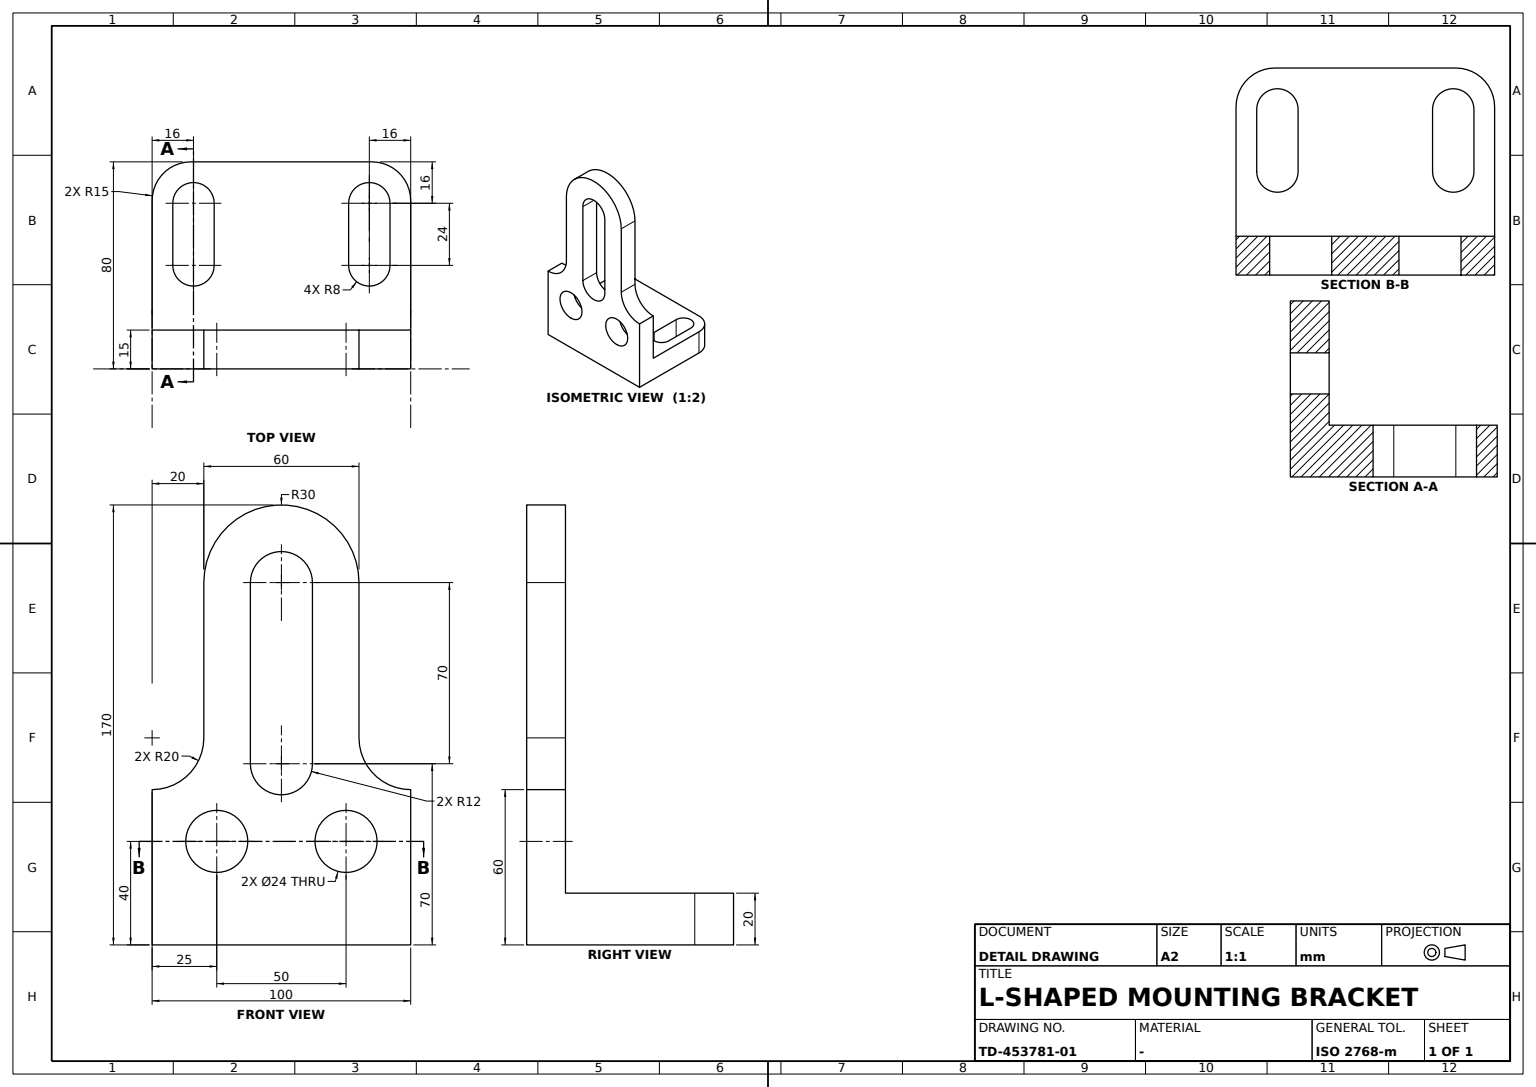
ISO-10303-21;
HEADER;
FILE_DESCRIPTION((''),'2;1');
FILE_NAME('','',(''),(''),'','','');
FILE_SCHEMA(('AUTOMOTIVE_DESIGN'));
ENDSEC;
DATA;
#1=APPLICATION_CONTEXT('');
#2=PRODUCT_CONTEXT('',#1,'mechanical');
#3=PRODUCT('','','',(#2));
#4=PRODUCT_DEFINITION_FORMATION('','',#3);
#5=PRODUCT_DEFINITION_CONTEXT('',#1,'design');
#6=PRODUCT_DEFINITION('','',#4,#5);
#7=PRODUCT_DEFINITION_SHAPE('','',#6);
#8=(LENGTH_UNIT()NAMED_UNIT(*)SI_UNIT(.MILLI.,.METRE.));
#9=(NAMED_UNIT(*)PLANE_ANGLE_UNIT()SI_UNIT($,.RADIAN.));
#10=(NAMED_UNIT(*)SI_UNIT($,.STERADIAN.)SOLID_ANGLE_UNIT());
#11=UNCERTAINTY_MEASURE_WITH_UNIT(LENGTH_MEASURE(0.005),#8,'distance_accuracy_value','');
#12=(GEOMETRIC_REPRESENTATION_CONTEXT(3)GLOBAL_UNCERTAINTY_ASSIGNED_CONTEXT((#11))GLOBAL_UNIT_ASSIGNED_CONTEXT((#8,#9,#10))REPRESENTATION_CONTEXT('',''));
#13=CARTESIAN_POINT('',(-12.,0.,130.));
#14=VERTEX_POINT('',#13);
#15=CARTESIAN_POINT('',(-12.,0.,60.));
#16=VERTEX_POINT('',#15);
#17=DIRECTION('',(0.,0.,-1.));
#18=VECTOR('',#17,1000.);
#19=LINE('',#13,#18);
#20=EDGE_CURVE('',#14,#16,#19,.T.);
#21=ORIENTED_EDGE('',*,*,#20,.T.);
#22=CARTESIAN_POINT('',(-12.,15.,60.));
#23=VERTEX_POINT('',#22);
#24=CARTESIAN_POINT('',(-12.,7.5,60.));
#25=DIRECTION('',(0.,-1.,0.));
#26=VECTOR('',#25,1000.);
#27=LINE('',#24,#26);
#28=EDGE_CURVE('',#16,#23,#27,.F.);
#29=ORIENTED_EDGE('',*,*,#28,.T.);
#30=CARTESIAN_POINT('',(-12.,15.,130.));
#31=VERTEX_POINT('',#30);
#32=LINE('',#30,#18);
#33=EDGE_CURVE('',#31,#23,#32,.T.);
#34=ORIENTED_EDGE('',*,*,#33,.F.);
#35=CARTESIAN_POINT('',(-12.,7.5,130.));
#36=LINE('',#35,#26);
#37=EDGE_CURVE('',#14,#31,#36,.F.);
#38=ORIENTED_EDGE('',*,*,#37,.F.);
#39=EDGE_LOOP('',(#21,#29,#34,#38));
#40=FACE_BOUND('',#39,.T.);
#41=DIRECTION('',(1.,0.,0.));
#42=AXIS2_PLACEMENT_3D('',#13,#41,#17);
#43=PLANE('',#42);
#44=ADVANCED_FACE('',(#40),#43,.T.);
#45=CARTESIAN_POINT('',(26.,40.,-10.));
#46=VERTEX_POINT('',#45);
#47=CARTESIAN_POINT('',(42.,40.,-10.));
#48=VERTEX_POINT('',#47);
#49=CARTESIAN_POINT('',(34.,40.,-10.));
#50=DIRECTION('',(0.,0.,1.));
#51=AXIS2_PLACEMENT_3D('',#49,#50,#41);
#52=CIRCLE('',#51,8.);
#53=EDGE_CURVE('',#46,#48,#52,.T.);
#54=ORIENTED_EDGE('',*,*,#53,.T.);
#55=CARTESIAN_POINT('',(42.,64.,-10.));
#56=VERTEX_POINT('',#55);
#57=CARTESIAN_POINT('',(42.,0.,-10.));
#58=DIRECTION('',(0.,1.,0.));
#59=VECTOR('',#58,1000.);
#60=LINE('',#57,#59);
#61=EDGE_CURVE('',#48,#56,#60,.T.);
#62=ORIENTED_EDGE('',*,*,#61,.T.);
#63=CARTESIAN_POINT('',(26.,64.,-10.));
#64=VERTEX_POINT('',#63);
#65=CARTESIAN_POINT('',(34.,64.,-10.));
#66=AXIS2_PLACEMENT_3D('',#65,#50,#41);
#67=CIRCLE('',#66,8.);
#68=EDGE_CURVE('',#56,#64,#67,.T.);
#69=ORIENTED_EDGE('',*,*,#68,.T.);
#70=CARTESIAN_POINT('',(26.,0.,-10.));
#71=LINE('',#70,#59);
#72=EDGE_CURVE('',#46,#64,#71,.T.);
#73=ORIENTED_EDGE('',*,*,#72,.F.);
#74=EDGE_LOOP('',(#54,#62,#69,#73));
#75=FACE_BOUND('',#74,.T.);
#76=CARTESIAN_POINT('',(-50.,0.,-10.));
#77=VERTEX_POINT('',#76);
#78=CARTESIAN_POINT('',(-50.,65.,-10.));
#79=VERTEX_POINT('',#78);
#80=LINE('',#76,#59);
#81=EDGE_CURVE('',#77,#79,#80,.T.);
#82=ORIENTED_EDGE('',*,*,#81,.T.);
#83=CARTESIAN_POINT('',(-35.,80.,-10.));
#84=VERTEX_POINT('',#83);
#85=CARTESIAN_POINT('',(-35.,65.,-10.));
#86=AXIS2_PLACEMENT_3D('',#85,#50,#41);
#87=CIRCLE('',#86,15.);
#88=EDGE_CURVE('',#84,#79,#87,.T.);
#89=ORIENTED_EDGE('',*,*,#88,.F.);
#90=CARTESIAN_POINT('',(35.,80.,-10.));
#91=VERTEX_POINT('',#90);
#92=CARTESIAN_POINT('',(0.,80.,-10.));
#93=DIRECTION('',(-1.,0.,0.));
#94=VECTOR('',#93,1000.);
#95=LINE('',#92,#94);
#96=EDGE_CURVE('',#91,#84,#95,.T.);
#97=ORIENTED_EDGE('',*,*,#96,.F.);
#98=CARTESIAN_POINT('',(50.,65.,-10.));
#99=VERTEX_POINT('',#98);
#100=CARTESIAN_POINT('',(35.,65.,-10.));
#101=AXIS2_PLACEMENT_3D('',#100,#50,#41);
#102=CIRCLE('',#101,15.);
#103=EDGE_CURVE('',#99,#91,#102,.T.);
#104=ORIENTED_EDGE('',*,*,#103,.F.);
#105=CARTESIAN_POINT('',(50.,0.,-10.));
#106=VERTEX_POINT('',#105);
#107=LINE('',#105,#26);
#108=EDGE_CURVE('',#99,#106,#107,.T.);
#109=ORIENTED_EDGE('',*,*,#108,.T.);
#110=CARTESIAN_POINT('',(0.,0.,-10.));
#111=VECTOR('',#41,1000.);
#112=LINE('',#110,#111);
#113=EDGE_CURVE('',#77,#106,#112,.T.);
#114=ORIENTED_EDGE('',*,*,#113,.F.);
#115=EDGE_LOOP('',(#82,#89,#97,#104,#109,#114));
#116=FACE_BOUND('',#115,.T.);
#117=CARTESIAN_POINT('',(-26.,40.,-10.));
#118=VERTEX_POINT('',#117);
#119=CARTESIAN_POINT('',(-26.,64.,-10.));
#120=VERTEX_POINT('',#119);
#121=CARTESIAN_POINT('',(-26.,0.,-10.));
#122=LINE('',#121,#59);
#123=EDGE_CURVE('',#118,#120,#122,.T.);
#124=ORIENTED_EDGE('',*,*,#123,.T.);
#125=CARTESIAN_POINT('',(-42.,64.,-10.));
#126=VERTEX_POINT('',#125);
#127=CARTESIAN_POINT('',(-34.,64.,-10.));
#128=AXIS2_PLACEMENT_3D('',#127,#50,#41);
#129=CIRCLE('',#128,8.);
#130=EDGE_CURVE('',#120,#126,#129,.T.);
#131=ORIENTED_EDGE('',*,*,#130,.T.);
#132=CARTESIAN_POINT('',(-42.,40.,-10.));
#133=VERTEX_POINT('',#132);
#134=CARTESIAN_POINT('',(-42.,0.,-10.));
#135=LINE('',#134,#59);
#136=EDGE_CURVE('',#133,#126,#135,.T.);
#137=ORIENTED_EDGE('',*,*,#136,.F.);
#138=CARTESIAN_POINT('',(-34.,40.,-10.));
#139=AXIS2_PLACEMENT_3D('',#138,#50,#41);
#140=CIRCLE('',#139,8.);
#141=EDGE_CURVE('',#133,#118,#140,.T.);
#142=ORIENTED_EDGE('',*,*,#141,.T.);
#143=EDGE_LOOP('',(#124,#131,#137,#142));
#144=FACE_BOUND('',#143,.T.);
#145=AXIS2_PLACEMENT_3D('',#110,#50,#58);
#146=PLANE('',#145);
#147=ADVANCED_FACE('',(#75,#116,#144),#146,.F.);
#148=ORIENTED_EDGE('',*,*,#37,.T.);
#149=CARTESIAN_POINT('',(12.,15.,130.));
#150=VERTEX_POINT('',#149);
#151=CARTESIAN_POINT('',(0.,15.,130.));
#152=AXIS2_PLACEMENT_3D('',#151,#25,#17);
#153=CIRCLE('',#152,12.);
#154=EDGE_CURVE('',#150,#31,#153,.T.);
#155=ORIENTED_EDGE('',*,*,#154,.F.);
#156=CARTESIAN_POINT('',(12.,0.,130.));
#157=VERTEX_POINT('',#156);
#158=CARTESIAN_POINT('',(12.,7.5,130.));
#159=LINE('',#158,#26);
#160=EDGE_CURVE('',#157,#150,#159,.F.);
#161=ORIENTED_EDGE('',*,*,#160,.F.);
#162=CARTESIAN_POINT('',(0.,0.,130.));
#163=AXIS2_PLACEMENT_3D('',#162,#25,#17);
#164=CIRCLE('',#163,12.);
#165=EDGE_CURVE('',#157,#14,#164,.T.);
#166=ORIENTED_EDGE('',*,*,#165,.T.);
#167=EDGE_LOOP('',(#148,#155,#161,#166));
#168=FACE_BOUND('',#167,.T.);
#169=CARTESIAN_POINT('',(0.,7.5,130.));
#170=AXIS2_PLACEMENT_3D('',#169,#25,#41);
#171=CYLINDRICAL_SURFACE('',#170,12.);
#172=ADVANCED_FACE('',(#168),#171,.F.);
#173=CARTESIAN_POINT('',(-26.,40.,10.));
#174=VERTEX_POINT('',#173);
#175=CARTESIAN_POINT('',(-26.,40.,0.));
#176=VECTOR('',#50,1000.);
#177=LINE('',#175,#176);
#178=EDGE_CURVE('',#118,#174,#177,.T.);
#179=ORIENTED_EDGE('',*,*,#178,.F.);
#180=ORIENTED_EDGE('',*,*,#141,.F.);
#181=CARTESIAN_POINT('',(-42.,40.,10.));
#182=VERTEX_POINT('',#181);
#183=CARTESIAN_POINT('',(-42.,40.,0.));
#184=LINE('',#183,#176);
#185=EDGE_CURVE('',#133,#182,#184,.T.);
#186=ORIENTED_EDGE('',*,*,#185,.T.);
#187=CARTESIAN_POINT('',(-34.,40.,10.));
#188=AXIS2_PLACEMENT_3D('',#187,#50,#41);
#189=CIRCLE('',#188,8.);
#190=EDGE_CURVE('',#182,#174,#189,.T.);
#191=ORIENTED_EDGE('',*,*,#190,.T.);
#192=EDGE_LOOP('',(#179,#180,#186,#191));
#193=FACE_BOUND('',#192,.T.);
#194=CARTESIAN_POINT('',(-34.,40.,0.));
#195=AXIS2_PLACEMENT_3D('',#194,#50,#58);
#196=CYLINDRICAL_SURFACE('',#195,8.);
#197=ADVANCED_FACE('',(#193),#196,.F.);
#198=CARTESIAN_POINT('',(42.,40.,10.));
#199=VERTEX_POINT('',#198);
#200=CARTESIAN_POINT('',(42.,40.,0.));
#201=LINE('',#200,#176);
#202=EDGE_CURVE('',#48,#199,#201,.T.);
#203=ORIENTED_EDGE('',*,*,#202,.F.);
#204=ORIENTED_EDGE('',*,*,#53,.F.);
#205=CARTESIAN_POINT('',(26.,40.,10.));
#206=VERTEX_POINT('',#205);
#207=CARTESIAN_POINT('',(26.,40.,0.));
#208=LINE('',#207,#176);
#209=EDGE_CURVE('',#46,#206,#208,.T.);
#210=ORIENTED_EDGE('',*,*,#209,.T.);
#211=CARTESIAN_POINT('',(34.,40.,10.));
#212=AXIS2_PLACEMENT_3D('',#211,#50,#41);
#213=CIRCLE('',#212,8.);
#214=EDGE_CURVE('',#206,#199,#213,.T.);
#215=ORIENTED_EDGE('',*,*,#214,.T.);
#216=EDGE_LOOP('',(#203,#204,#210,#215));
#217=FACE_BOUND('',#216,.T.);
#218=CARTESIAN_POINT('',(34.,40.,0.));
#219=AXIS2_PLACEMENT_3D('',#218,#50,#58);
#220=CYLINDRICAL_SURFACE('',#219,8.);
#221=ADVANCED_FACE('',(#217),#220,.F.);
#222=CARTESIAN_POINT('',(-30.,0.,70.));
#223=VERTEX_POINT('',#222);
#224=CARTESIAN_POINT('',(-30.,0.,130.));
#225=VERTEX_POINT('',#224);
#226=CARTESIAN_POINT('',(-30.,0.,50.));
#227=LINE('',#226,#176);
#228=EDGE_CURVE('',#223,#225,#227,.T.);
#229=ORIENTED_EDGE('',*,*,#228,.T.);
#230=CARTESIAN_POINT('',(-30.,15.,130.));
#231=VERTEX_POINT('',#230);
#232=CARTESIAN_POINT('',(-30.,7.5,130.));
#233=LINE('',#232,#26);
#234=EDGE_CURVE('',#225,#231,#233,.F.);
#235=ORIENTED_EDGE('',*,*,#234,.T.);
#236=CARTESIAN_POINT('',(-30.,15.,70.));
#237=VERTEX_POINT('',#236);
#238=CARTESIAN_POINT('',(-30.,15.,50.));
#239=LINE('',#238,#176);
#240=EDGE_CURVE('',#237,#231,#239,.T.);
#241=ORIENTED_EDGE('',*,*,#240,.F.);
#242=CARTESIAN_POINT('',(-30.,7.5,70.));
#243=LINE('',#242,#26);
#244=EDGE_CURVE('',#223,#237,#243,.F.);
#245=ORIENTED_EDGE('',*,*,#244,.F.);
#246=EDGE_LOOP('',(#229,#235,#241,#245));
#247=FACE_BOUND('',#246,.T.);
#248=AXIS2_PLACEMENT_3D('',#226,#93,#50);
#249=PLANE('',#248);
#250=ADVANCED_FACE('',(#247),#249,.T.);
#251=CARTESIAN_POINT('',(30.,0.,130.));
#252=VERTEX_POINT('',#251);
#253=CARTESIAN_POINT('',(30.,15.,130.));
#254=VERTEX_POINT('',#253);
#255=CARTESIAN_POINT('',(30.,7.5,130.));
#256=LINE('',#255,#26);
#257=EDGE_CURVE('',#252,#254,#256,.F.);
#258=ORIENTED_EDGE('',*,*,#257,.F.);
#259=CARTESIAN_POINT('',(30.,0.,70.));
#260=VERTEX_POINT('',#259);
#261=LINE('',#251,#18);
#262=EDGE_CURVE('',#252,#260,#261,.T.);
#263=ORIENTED_EDGE('',*,*,#262,.T.);
#264=CARTESIAN_POINT('',(30.,15.,70.));
#265=VERTEX_POINT('',#264);
#266=CARTESIAN_POINT('',(30.,7.5,70.));
#267=LINE('',#266,#59);
#268=EDGE_CURVE('',#260,#265,#267,.T.);
#269=ORIENTED_EDGE('',*,*,#268,.T.);
#270=LINE('',#253,#18);
#271=EDGE_CURVE('',#254,#265,#270,.T.);
#272=ORIENTED_EDGE('',*,*,#271,.F.);
#273=EDGE_LOOP('',(#258,#263,#269,#272));
#274=FACE_BOUND('',#273,.T.);
#275=AXIS2_PLACEMENT_3D('',#251,#41,#17);
#276=PLANE('',#275);
#277=ADVANCED_FACE('',(#274),#276,.T.);
#278=CARTESIAN_POINT('',(12.,0.,60.));
#279=VERTEX_POINT('',#278);
#280=CARTESIAN_POINT('',(12.,15.,60.));
#281=VERTEX_POINT('',#280);
#282=CARTESIAN_POINT('',(12.,7.5,60.));
#283=LINE('',#282,#26);
#284=EDGE_CURVE('',#279,#281,#283,.F.);
#285=ORIENTED_EDGE('',*,*,#284,.F.);
#286=LINE('',#156,#18);
#287=EDGE_CURVE('',#157,#279,#286,.T.);
#288=ORIENTED_EDGE('',*,*,#287,.F.);
#289=ORIENTED_EDGE('',*,*,#160,.T.);
#290=LINE('',#149,#18);
#291=EDGE_CURVE('',#150,#281,#290,.T.);
#292=ORIENTED_EDGE('',*,*,#291,.T.);
#293=EDGE_LOOP('',(#285,#288,#289,#292));
#294=FACE_BOUND('',#293,.T.);
#295=AXIS2_PLACEMENT_3D('',#156,#41,#17);
#296=PLANE('',#295);
#297=ADVANCED_FACE('',(#294),#296,.F.);
#298=CARTESIAN_POINT('',(-26.,64.,10.));
#299=VERTEX_POINT('',#298);
#300=CARTESIAN_POINT('',(-42.,64.,10.));
#301=VERTEX_POINT('',#300);
#302=CARTESIAN_POINT('',(-34.,64.,10.));
#303=AXIS2_PLACEMENT_3D('',#302,#50,#41);
#304=CIRCLE('',#303,8.);
#305=EDGE_CURVE('',#299,#301,#304,.T.);
#306=ORIENTED_EDGE('',*,*,#305,.T.);
#307=CARTESIAN_POINT('',(-42.,64.,0.));
#308=LINE('',#307,#176);
#309=EDGE_CURVE('',#126,#301,#308,.T.);
#310=ORIENTED_EDGE('',*,*,#309,.F.);
#311=ORIENTED_EDGE('',*,*,#130,.F.);
#312=CARTESIAN_POINT('',(-26.,64.,0.));
#313=LINE('',#312,#176);
#314=EDGE_CURVE('',#120,#299,#313,.T.);
#315=ORIENTED_EDGE('',*,*,#314,.T.);
#316=EDGE_LOOP('',(#306,#310,#311,#315));
#317=FACE_BOUND('',#316,.T.);
#318=CARTESIAN_POINT('',(-34.,64.,0.));
#319=AXIS2_PLACEMENT_3D('',#318,#50,#58);
#320=CYLINDRICAL_SURFACE('',#319,8.);
#321=ADVANCED_FACE('',(#317),#320,.F.);
#322=ORIENTED_EDGE('',*,*,#136,.T.);
#323=ORIENTED_EDGE('',*,*,#309,.T.);
#324=CARTESIAN_POINT('',(-42.,0.,10.));
#325=LINE('',#324,#59);
#326=EDGE_CURVE('',#182,#301,#325,.T.);
#327=ORIENTED_EDGE('',*,*,#326,.F.);
#328=ORIENTED_EDGE('',*,*,#185,.F.);
#329=EDGE_LOOP('',(#322,#323,#327,#328));
#330=FACE_BOUND('',#329,.T.);
#331=AXIS2_PLACEMENT_3D('',#183,#41,#58);
#332=PLANE('',#331);
#333=ADVANCED_FACE('',(#330),#332,.T.);
#334=CARTESIAN_POINT('',(25.,15.,18.));
#335=VERTEX_POINT('',#334);
#336=CARTESIAN_POINT('',(25.,15.,30.));
#337=AXIS2_PLACEMENT_3D('',#336,#25,#17);
#338=CIRCLE('',#337,12.);
#339=EDGE_CURVE('',#335,#335,#338,.T.);
#340=ORIENTED_EDGE('',*,*,#339,.T.);
#341=EDGE_LOOP('',(#340));
#342=FACE_BOUND('',#341,.T.);
#343=CARTESIAN_POINT('',(0.,15.,60.));
#344=AXIS2_PLACEMENT_3D('',#343,#25,#17);
#345=CIRCLE('',#344,12.);
#346=EDGE_CURVE('',#23,#281,#345,.T.);
#347=ORIENTED_EDGE('',*,*,#346,.T.);
#348=ORIENTED_EDGE('',*,*,#291,.F.);
#349=ORIENTED_EDGE('',*,*,#154,.T.);
#350=ORIENTED_EDGE('',*,*,#33,.T.);
#351=EDGE_LOOP('',(#347,#348,#349,#350));
#352=FACE_BOUND('',#351,.T.);
#353=CARTESIAN_POINT('',(-25.,15.,18.));
#354=VERTEX_POINT('',#353);
#355=CARTESIAN_POINT('',(-25.,15.,30.));
#356=AXIS2_PLACEMENT_3D('',#355,#25,#17);
#357=CIRCLE('',#356,12.);
#358=EDGE_CURVE('',#354,#354,#357,.T.);
#359=ORIENTED_EDGE('',*,*,#358,.T.);
#360=EDGE_LOOP('',(#359));
#361=FACE_BOUND('',#360,.T.);
#362=ORIENTED_EDGE('',*,*,#240,.T.);
#363=CIRCLE('',#152,30.);
#364=EDGE_CURVE('',#254,#231,#363,.T.);
#365=ORIENTED_EDGE('',*,*,#364,.F.);
#366=ORIENTED_EDGE('',*,*,#271,.T.);
#367=CARTESIAN_POINT('',(50.,15.,50.));
#368=VERTEX_POINT('',#367);
#369=CARTESIAN_POINT('',(50.,15.,70.));
#370=AXIS2_PLACEMENT_3D('',#369,#25,#17);
#371=CIRCLE('',#370,20.);
#372=EDGE_CURVE('',#265,#368,#371,.T.);
#373=ORIENTED_EDGE('',*,*,#372,.T.);
#374=CARTESIAN_POINT('',(50.,15.,10.));
#375=VERTEX_POINT('',#374);
#376=CARTESIAN_POINT('',(50.,15.,0.));
#377=LINE('',#376,#18);
#378=EDGE_CURVE('',#368,#375,#377,.T.);
#379=ORIENTED_EDGE('',*,*,#378,.T.);
#380=CARTESIAN_POINT('',(-50.,15.,10.));
#381=VERTEX_POINT('',#380);
#382=CARTESIAN_POINT('',(0.,15.,10.));
#383=LINE('',#382,#111);
#384=EDGE_CURVE('',#381,#375,#383,.T.);
#385=ORIENTED_EDGE('',*,*,#384,.F.);
#386=CARTESIAN_POINT('',(-50.,15.,50.));
#387=VERTEX_POINT('',#386);
#388=CARTESIAN_POINT('',(-50.,15.,0.));
#389=LINE('',#388,#176);
#390=EDGE_CURVE('',#381,#387,#389,.T.);
#391=ORIENTED_EDGE('',*,*,#390,.T.);
#392=CARTESIAN_POINT('',(-50.,15.,70.));
#393=AXIS2_PLACEMENT_3D('',#392,#25,#17);
#394=CIRCLE('',#393,20.);
#395=EDGE_CURVE('',#387,#237,#394,.T.);
#396=ORIENTED_EDGE('',*,*,#395,.T.);
#397=EDGE_LOOP('',(#362,#365,#366,#373,#379,#385,#391,#396));
#398=FACE_BOUND('',#397,.T.);
#399=CARTESIAN_POINT('',(0.,15.,0.));
#400=AXIS2_PLACEMENT_3D('',#399,#25,#41);
#401=PLANE('',#400);
#402=ADVANCED_FACE('',(#342,#352,#361,#398),#401,.F.);
#403=CARTESIAN_POINT('',(42.,64.,10.));
#404=VERTEX_POINT('',#403);
#405=CARTESIAN_POINT('',(42.,64.,0.));
#406=LINE('',#405,#176);
#407=EDGE_CURVE('',#56,#404,#406,.T.);
#408=ORIENTED_EDGE('',*,*,#407,.F.);
#409=ORIENTED_EDGE('',*,*,#61,.F.);
#410=ORIENTED_EDGE('',*,*,#202,.T.);
#411=CARTESIAN_POINT('',(42.,0.,10.));
#412=LINE('',#411,#59);
#413=EDGE_CURVE('',#199,#404,#412,.T.);
#414=ORIENTED_EDGE('',*,*,#413,.T.);
#415=EDGE_LOOP('',(#408,#409,#410,#414));
#416=FACE_BOUND('',#415,.T.);
#417=AXIS2_PLACEMENT_3D('',#200,#41,#58);
#418=PLANE('',#417);
#419=ADVANCED_FACE('',(#416),#418,.F.);
#420=ORIENTED_EDGE('',*,*,#358,.F.);
#421=EDGE_LOOP('',(#420));
#422=FACE_BOUND('',#421,.T.);
#423=CARTESIAN_POINT('',(-25.,0.,18.));
#424=VERTEX_POINT('',#423);
#425=CARTESIAN_POINT('',(-25.,0.,30.));
#426=AXIS2_PLACEMENT_3D('',#425,#25,#17);
#427=CIRCLE('',#426,12.);
#428=EDGE_CURVE('',#424,#424,#427,.T.);
#429=ORIENTED_EDGE('',*,*,#428,.T.);
#430=EDGE_LOOP('',(#429));
#431=FACE_BOUND('',#430,.T.);
#432=CARTESIAN_POINT('',(-25.,7.5,30.));
#433=AXIS2_PLACEMENT_3D('',#432,#25,#41);
#434=CYLINDRICAL_SURFACE('',#433,12.);
#435=ADVANCED_FACE('',(#422,#431),#434,.F.);
#436=CARTESIAN_POINT('',(50.,0.,50.));
#437=VERTEX_POINT('',#436);
#438=CARTESIAN_POINT('',(50.,0.,0.));
#439=LINE('',#438,#176);
#440=EDGE_CURVE('',#106,#437,#439,.T.);
#441=ORIENTED_EDGE('',*,*,#440,.T.);
#442=CARTESIAN_POINT('',(50.,0.,70.));
#443=AXIS2_PLACEMENT_3D('',#442,#25,#17);
#444=CIRCLE('',#443,20.);
#445=EDGE_CURVE('',#260,#437,#444,.T.);
#446=ORIENTED_EDGE('',*,*,#445,.F.);
#447=ORIENTED_EDGE('',*,*,#262,.F.);
#448=CIRCLE('',#163,30.);
#449=EDGE_CURVE('',#252,#225,#448,.T.);
#450=ORIENTED_EDGE('',*,*,#449,.T.);
#451=ORIENTED_EDGE('',*,*,#228,.F.);
#452=CARTESIAN_POINT('',(-50.,0.,50.));
#453=VERTEX_POINT('',#452);
#454=CARTESIAN_POINT('',(-50.,0.,70.));
#455=AXIS2_PLACEMENT_3D('',#454,#25,#17);
#456=CIRCLE('',#455,20.);
#457=EDGE_CURVE('',#453,#223,#456,.T.);
#458=ORIENTED_EDGE('',*,*,#457,.F.);
#459=CARTESIAN_POINT('',(-50.,0.,0.));
#460=LINE('',#459,#176);
#461=EDGE_CURVE('',#77,#453,#460,.T.);
#462=ORIENTED_EDGE('',*,*,#461,.F.);
#463=ORIENTED_EDGE('',*,*,#113,.T.);
#464=EDGE_LOOP('',(#441,#446,#447,#450,#451,#458,#462,#463));
#465=FACE_BOUND('',#464,.T.);
#466=CARTESIAN_POINT('',(25.,0.,18.));
#467=VERTEX_POINT('',#466);
#468=CARTESIAN_POINT('',(25.,0.,30.));
#469=AXIS2_PLACEMENT_3D('',#468,#25,#17);
#470=CIRCLE('',#469,12.);
#471=EDGE_CURVE('',#467,#467,#470,.T.);
#472=ORIENTED_EDGE('',*,*,#471,.F.);
#473=EDGE_LOOP('',(#472));
#474=FACE_BOUND('',#473,.T.);
#475=ORIENTED_EDGE('',*,*,#428,.F.);
#476=EDGE_LOOP('',(#475));
#477=FACE_BOUND('',#476,.T.);
#478=CARTESIAN_POINT('',(0.,0.,60.));
#479=AXIS2_PLACEMENT_3D('',#478,#25,#17);
#480=CIRCLE('',#479,12.);
#481=EDGE_CURVE('',#16,#279,#480,.T.);
#482=ORIENTED_EDGE('',*,*,#481,.F.);
#483=ORIENTED_EDGE('',*,*,#20,.F.);
#484=ORIENTED_EDGE('',*,*,#165,.F.);
#485=ORIENTED_EDGE('',*,*,#287,.T.);
#486=EDGE_LOOP('',(#482,#483,#484,#485));
#487=FACE_BOUND('',#486,.T.);
#488=AXIS2_PLACEMENT_3D('',#459,#25,#41);
#489=PLANE('',#488);
#490=ADVANCED_FACE('',(#465,#474,#477,#487),#489,.T.);
#491=ORIENTED_EDGE('',*,*,#88,.T.);
#492=CARTESIAN_POINT('',(-50.,65.,10.));
#493=VERTEX_POINT('',#492);
#494=CARTESIAN_POINT('',(-50.,65.,0.));
#495=LINE('',#494,#176);
#496=EDGE_CURVE('',#79,#493,#495,.T.);
#497=ORIENTED_EDGE('',*,*,#496,.T.);
#498=CARTESIAN_POINT('',(-35.,80.,10.));
#499=VERTEX_POINT('',#498);
#500=CARTESIAN_POINT('',(-35.,65.,10.));
#501=AXIS2_PLACEMENT_3D('',#500,#50,#41);
#502=CIRCLE('',#501,15.);
#503=EDGE_CURVE('',#499,#493,#502,.T.);
#504=ORIENTED_EDGE('',*,*,#503,.F.);
#505=CARTESIAN_POINT('',(-35.,80.,0.));
#506=LINE('',#505,#176);
#507=EDGE_CURVE('',#84,#499,#506,.T.);
#508=ORIENTED_EDGE('',*,*,#507,.F.);
#509=EDGE_LOOP('',(#491,#497,#504,#508));
#510=FACE_BOUND('',#509,.T.);
#511=CARTESIAN_POINT('',(-35.,65.,0.));
#512=AXIS2_PLACEMENT_3D('',#511,#50,#93);
#513=CYLINDRICAL_SURFACE('',#512,15.);
#514=ADVANCED_FACE('',(#510),#513,.T.);
#515=CARTESIAN_POINT('',(50.,65.,10.));
#516=VERTEX_POINT('',#515);
#517=CARTESIAN_POINT('',(50.,65.,0.));
#518=LINE('',#517,#176);
#519=EDGE_CURVE('',#99,#516,#518,.T.);
#520=ORIENTED_EDGE('',*,*,#519,.T.);
#521=CARTESIAN_POINT('',(50.,0.,10.));
#522=LINE('',#521,#26);
#523=EDGE_CURVE('',#516,#375,#522,.T.);
#524=ORIENTED_EDGE('',*,*,#523,.T.);
#525=ORIENTED_EDGE('',*,*,#378,.F.);
#526=LINE('',#436,#59);
#527=EDGE_CURVE('',#437,#368,#526,.T.);
#528=ORIENTED_EDGE('',*,*,#527,.F.);
#529=ORIENTED_EDGE('',*,*,#440,.F.);
#530=ORIENTED_EDGE('',*,*,#108,.F.);
#531=EDGE_LOOP('',(#520,#524,#525,#528,#529,#530));
#532=FACE_BOUND('',#531,.T.);
#533=CARTESIAN_POINT('',(50.,80.,0.));
#534=AXIS2_PLACEMENT_3D('',#533,#93,#25);
#535=PLANE('',#534);
#536=ADVANCED_FACE('',(#532),#535,.F.);
#537=CARTESIAN_POINT('',(-50.,0.,10.));
#538=LINE('',#537,#59);
#539=EDGE_CURVE('',#381,#493,#538,.T.);
#540=ORIENTED_EDGE('',*,*,#539,.T.);
#541=ORIENTED_EDGE('',*,*,#496,.F.);
#542=ORIENTED_EDGE('',*,*,#81,.F.);
#543=ORIENTED_EDGE('',*,*,#461,.T.);
#544=LINE('',#452,#26);
#545=EDGE_CURVE('',#453,#387,#544,.F.);
#546=ORIENTED_EDGE('',*,*,#545,.T.);
#547=ORIENTED_EDGE('',*,*,#390,.F.);
#548=EDGE_LOOP('',(#540,#541,#542,#543,#546,#547));
#549=FACE_BOUND('',#548,.T.);
#550=AXIS2_PLACEMENT_3D('',#459,#41,#58);
#551=PLANE('',#550);
#552=ADVANCED_FACE('',(#549),#551,.F.);
#553=CARTESIAN_POINT('',(26.,64.,10.));
#554=VERTEX_POINT('',#553);
#555=CARTESIAN_POINT('',(26.,64.,0.));
#556=LINE('',#555,#176);
#557=EDGE_CURVE('',#64,#554,#556,.T.);
#558=ORIENTED_EDGE('',*,*,#557,.T.);
#559=CARTESIAN_POINT('',(26.,0.,10.));
#560=LINE('',#559,#59);
#561=EDGE_CURVE('',#206,#554,#560,.T.);
#562=ORIENTED_EDGE('',*,*,#561,.F.);
#563=ORIENTED_EDGE('',*,*,#209,.F.);
#564=ORIENTED_EDGE('',*,*,#72,.T.);
#565=EDGE_LOOP('',(#558,#562,#563,#564));
#566=FACE_BOUND('',#565,.T.);
#567=AXIS2_PLACEMENT_3D('',#207,#41,#58);
#568=PLANE('',#567);
#569=ADVANCED_FACE('',(#566),#568,.T.);
#570=ORIENTED_EDGE('',*,*,#284,.T.);
#571=ORIENTED_EDGE('',*,*,#346,.F.);
#572=ORIENTED_EDGE('',*,*,#28,.F.);
#573=ORIENTED_EDGE('',*,*,#481,.T.);
#574=EDGE_LOOP('',(#570,#571,#572,#573));
#575=FACE_BOUND('',#574,.T.);
#576=CARTESIAN_POINT('',(0.,7.5,60.));
#577=AXIS2_PLACEMENT_3D('',#576,#25,#41);
#578=CYLINDRICAL_SURFACE('',#577,12.);
#579=ADVANCED_FACE('',(#575),#578,.F.);
#580=ORIENTED_EDGE('',*,*,#364,.T.);
#581=ORIENTED_EDGE('',*,*,#234,.F.);
#582=ORIENTED_EDGE('',*,*,#449,.F.);
#583=ORIENTED_EDGE('',*,*,#257,.T.);
#584=EDGE_LOOP('',(#580,#581,#582,#583));
#585=FACE_BOUND('',#584,.T.);
#586=CYLINDRICAL_SURFACE('',#170,30.);
#587=ADVANCED_FACE('',(#585),#586,.T.);
#588=CARTESIAN_POINT('',(35.,80.,10.));
#589=VERTEX_POINT('',#588);
#590=CARTESIAN_POINT('',(0.,80.,10.));
#591=LINE('',#590,#94);
#592=EDGE_CURVE('',#589,#499,#591,.T.);
#593=ORIENTED_EDGE('',*,*,#592,.F.);
#594=CARTESIAN_POINT('',(35.,80.,0.));
#595=LINE('',#594,#176);
#596=EDGE_CURVE('',#91,#589,#595,.T.);
#597=ORIENTED_EDGE('',*,*,#596,.F.);
#598=ORIENTED_EDGE('',*,*,#96,.T.);
#599=ORIENTED_EDGE('',*,*,#507,.T.);
#600=EDGE_LOOP('',(#593,#597,#598,#599));
#601=FACE_BOUND('',#600,.T.);
#602=AXIS2_PLACEMENT_3D('',#533,#58,#93);
#603=PLANE('',#602);
#604=ADVANCED_FACE('',(#601),#603,.T.);
#605=ORIENTED_EDGE('',*,*,#372,.F.);
#606=ORIENTED_EDGE('',*,*,#268,.F.);
#607=ORIENTED_EDGE('',*,*,#445,.T.);
#608=ORIENTED_EDGE('',*,*,#527,.T.);
#609=EDGE_LOOP('',(#605,#606,#607,#608));
#610=FACE_BOUND('',#609,.T.);
#611=CARTESIAN_POINT('',(50.,7.5,70.));
#612=AXIS2_PLACEMENT_3D('',#611,#58,#17);
#613=CYLINDRICAL_SURFACE('',#612,20.);
#614=ADVANCED_FACE('',(#610),#613,.F.);
#615=ORIENTED_EDGE('',*,*,#545,.F.);
#616=ORIENTED_EDGE('',*,*,#457,.T.);
#617=ORIENTED_EDGE('',*,*,#244,.T.);
#618=ORIENTED_EDGE('',*,*,#395,.F.);
#619=EDGE_LOOP('',(#615,#616,#617,#618));
#620=FACE_BOUND('',#619,.T.);
#621=CARTESIAN_POINT('',(-50.,7.5,70.));
#622=AXIS2_PLACEMENT_3D('',#621,#25,#17);
#623=CYLINDRICAL_SURFACE('',#622,20.);
#624=ADVANCED_FACE('',(#620),#623,.F.);
#625=ORIENTED_EDGE('',*,*,#561,.T.);
#626=CARTESIAN_POINT('',(34.,64.,10.));
#627=AXIS2_PLACEMENT_3D('',#626,#50,#41);
#628=CIRCLE('',#627,8.);
#629=EDGE_CURVE('',#404,#554,#628,.T.);
#630=ORIENTED_EDGE('',*,*,#629,.F.);
#631=ORIENTED_EDGE('',*,*,#413,.F.);
#632=ORIENTED_EDGE('',*,*,#214,.F.);
#633=EDGE_LOOP('',(#625,#630,#631,#632));
#634=FACE_BOUND('',#633,.T.);
#635=ORIENTED_EDGE('',*,*,#384,.T.);
#636=ORIENTED_EDGE('',*,*,#523,.F.);
#637=CARTESIAN_POINT('',(35.,65.,10.));
#638=AXIS2_PLACEMENT_3D('',#637,#50,#41);
#639=CIRCLE('',#638,15.);
#640=EDGE_CURVE('',#516,#589,#639,.T.);
#641=ORIENTED_EDGE('',*,*,#640,.T.);
#642=ORIENTED_EDGE('',*,*,#592,.T.);
#643=ORIENTED_EDGE('',*,*,#503,.T.);
#644=ORIENTED_EDGE('',*,*,#539,.F.);
#645=EDGE_LOOP('',(#635,#636,#641,#642,#643,#644));
#646=FACE_BOUND('',#645,.T.);
#647=ORIENTED_EDGE('',*,*,#305,.F.);
#648=CARTESIAN_POINT('',(-26.,0.,10.));
#649=LINE('',#648,#59);
#650=EDGE_CURVE('',#174,#299,#649,.T.);
#651=ORIENTED_EDGE('',*,*,#650,.F.);
#652=ORIENTED_EDGE('',*,*,#190,.F.);
#653=ORIENTED_EDGE('',*,*,#326,.T.);
#654=EDGE_LOOP('',(#647,#651,#652,#653));
#655=FACE_BOUND('',#654,.T.);
#656=CARTESIAN_POINT('',(0.,0.,10.));
#657=AXIS2_PLACEMENT_3D('',#656,#50,#58);
#658=PLANE('',#657);
#659=ADVANCED_FACE('',(#634,#646,#655),#658,.T.);
#660=ORIENTED_EDGE('',*,*,#314,.F.);
#661=ORIENTED_EDGE('',*,*,#123,.F.);
#662=ORIENTED_EDGE('',*,*,#178,.T.);
#663=ORIENTED_EDGE('',*,*,#650,.T.);
#664=EDGE_LOOP('',(#660,#661,#662,#663));
#665=FACE_BOUND('',#664,.T.);
#666=AXIS2_PLACEMENT_3D('',#175,#41,#58);
#667=PLANE('',#666);
#668=ADVANCED_FACE('',(#665),#667,.F.);
#669=ORIENTED_EDGE('',*,*,#471,.T.);
#670=EDGE_LOOP('',(#669));
#671=FACE_BOUND('',#670,.T.);
#672=ORIENTED_EDGE('',*,*,#339,.F.);
#673=EDGE_LOOP('',(#672));
#674=FACE_BOUND('',#673,.T.);
#675=CARTESIAN_POINT('',(25.,7.5,30.));
#676=AXIS2_PLACEMENT_3D('',#675,#25,#41);
#677=CYLINDRICAL_SURFACE('',#676,12.);
#678=ADVANCED_FACE('',(#671,#674),#677,.F.);
#679=ORIENTED_EDGE('',*,*,#519,.F.);
#680=ORIENTED_EDGE('',*,*,#103,.T.);
#681=ORIENTED_EDGE('',*,*,#596,.T.);
#682=ORIENTED_EDGE('',*,*,#640,.F.);
#683=EDGE_LOOP('',(#679,#680,#681,#682));
#684=FACE_BOUND('',#683,.T.);
#685=CARTESIAN_POINT('',(35.,65.,0.));
#686=AXIS2_PLACEMENT_3D('',#685,#50,#58);
#687=CYLINDRICAL_SURFACE('',#686,15.);
#688=ADVANCED_FACE('',(#684),#687,.T.);
#689=ORIENTED_EDGE('',*,*,#629,.T.);
#690=ORIENTED_EDGE('',*,*,#557,.F.);
#691=ORIENTED_EDGE('',*,*,#68,.F.);
#692=ORIENTED_EDGE('',*,*,#407,.T.);
#693=EDGE_LOOP('',(#689,#690,#691,#692));
#694=FACE_BOUND('',#693,.T.);
#695=CARTESIAN_POINT('',(34.,64.,0.));
#696=AXIS2_PLACEMENT_3D('',#695,#50,#58);
#697=CYLINDRICAL_SURFACE('',#696,8.);
#698=ADVANCED_FACE('',(#694),#697,.F.);
#699=CLOSED_SHELL('',(#44,#147,#172,#197,#221,#250,#277,#297,#321,#333,#402,#419,#435,#490,#514,#536,#552,#569,#579,#587,#604,#614,#624,#659,#668,#678,#688,#698));
#700=MANIFOLD_SOLID_BREP('',#699);
#701=ADVANCED_BREP_SHAPE_REPRESENTATION('',(#700),#12);
#702=SHAPE_DEFINITION_REPRESENTATION(#7,#701);
ENDSEC;
END-ISO-10303-21;
